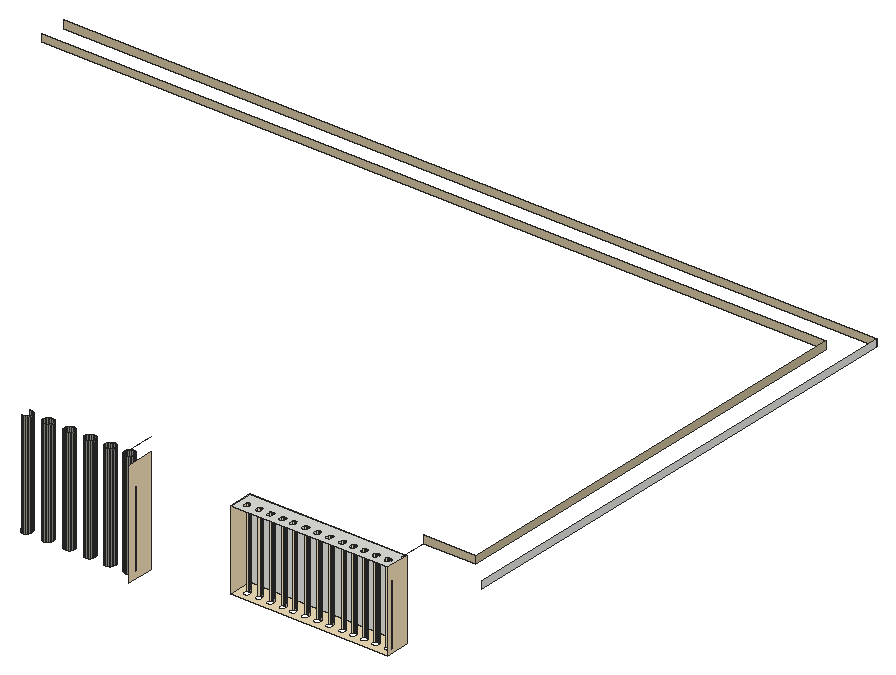
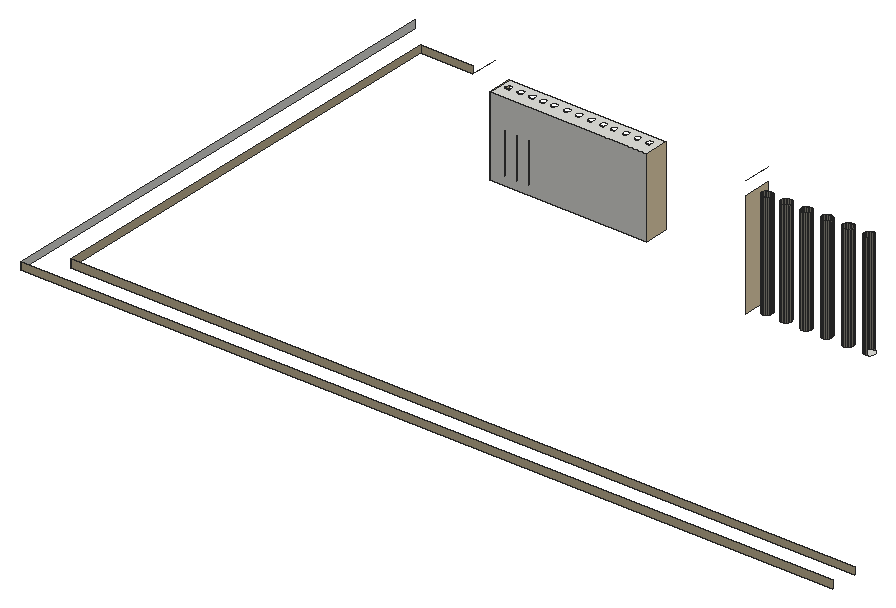
# SketchUp Ruby script. Lengths in inches.
U = 1.inch
M = Sketchup.active_model
def pt(a) = Geom::Point3d.new(a.map { |v| v * U })
def face(e, loops, mat)
  f = e.add_face(loops[0].map { |a| pt(a) })
  loops[1..].each { |l| e.add_face(l.map { |a| pt(a) }).erase! }
  f.material = f.back_material = mat if mat
  f
end
# faces: each face lists its corners as indices into pts; further lists are holes
def faces(e, pts, list, mat = nil) = list.each { |f| face(e, (f[0].is_a?(Array) ? f : [f]).map { |l| l.map { |i| pts[i] } }, mat) }
# xy, xz, yz: faces in a plane at the given z, y or x. An outline is a flat list of corners, or four numbers for a rectangle; further outlines are holes
def ring(l) = l.size == 4 ? [[l[0], l[1]], [l[2], l[1]], [l[2], l[3]], [l[0], l[3]]] : l.each_slice(2).to_a
def flat(e, list, mat, &to3) = list.each { |f| face(e, (f[0].is_a?(Array) ? f : [f]).map { |l| ring(l).map { |u, v| to3.(u, v) } }, mat) }
def xy(e, z, list, mat = nil) = flat(e, list, mat) { |x, y| [x, y, z] }
def xz(e, y, list, mat = nil) = flat(e, list, mat) { |x, z| [x, y, z] }
def yz(e, x, list, mat = nil) = flat(e, list, mat) { |y, z| [x, y, z] }
def lines(e, pts, list) = list.each { |a, b| e.add_line(pt(pts[a]), pt(pts[b])) }
# prism: a flat outline (further loops are holes) pulled along v
def prism(e, loops, v, mat = nil)
  f = face(e, loops, mat); d = Geom::Vector3d.new(v.map { |x| x * U })
  f.pushpull(f.normal.samedirection?(d) ? d.length : -d.length)
end
def box(e, o, s, mat = nil) = prism(e, [[o, [o[0] + s[0], o[1], o[2]], [o[0] + s[0], o[1] + s[1], o[2]], [o[0], o[1] + s[1], o[2]]]], [0, 0, s[2]], mat)
def at(x, y, z, deg = 0) = Geom::Transformation.translation(pt([x, y, z])) * Geom::Transformation.rotation(ORIGIN, Z_AXIS, deg.degrees)
def axes(o, x, y, z) = Geom::Transformation.new([*x, 0, *y, 0, *z, 0, *pt(o).to_a, 1])
def part(name) = M.definitions.add(name)
# library, detail: a bought-in or finely detailed component or shape, given as its bounding box
def library(name, o, s) = part(name).tap { |d| box(d.entities, o, s) }
def detail(e, o, s) = box(e.add_group.entities, o, s)
def put(e, d, t, mat = nil) = e.add_instance(d, t).tap { |i| i.material = mat if mat }
def group(e, t, mat = nil) = e.add_group.tap { |g| g.transformation = t; g.material = mat if mat }.entities
root = M.entities
M.materials.add("[Formica Graystone]").color = [149, 146, 135]
M.materials.add("[Quartz Light Brown]").color = [242, 223, 185]
M.materials.add("[Quartz Light Brown]2").color = [199, 184, 152]
xy(root,552.75,[[371.75,21.93,371.04,22.02,370.375,22.3,369.81,22.74,369.37,23.3,369.09,23.97,369,24.68,369.09,25.39,369.37,26.05,369.81,26.625,370.375,27.0625,371.04,27.34,371.75,27.43,372.46,27.34,373.125,27.0625,373.69,26.625,374.13,26.05,374.41,25.39,374.5,24.68,374.41,23.97,374.13,23.3,373.69,22.74,373.125,22.3,372.46,22.02],[383.125,21.93,382.41,22.02,381.75,22.3,381.18,22.74,380.74,23.3,380.47,23.97,380.375,24.68,380.47,25.39,380.74,26.05,381.18,26.625,381.75,27.0625,382.41,27.34,383.125,27.43,383.84,27.34,384.5,27.0625,385.07,26.625,385.51,26.05,385.78,25.39,385.875,24.68,385.78,23.97,385.51,23.3,385.07,22.74,384.5,22.3,383.84,22.02],[394.5,21.93,393.79,22.02,393.125,22.3,392.56,22.74,392.12,23.3,391.84,23.97,391.75,24.68,391.84,25.39,392.12,26.05,392.56,26.625,393.125,27.0625,393.79,27.34,394.5,27.43,395.21,27.34,395.875,27.0625,396.44,26.625,396.88,26.05,397.16,25.39,397.25,24.68,397.16,23.97,396.88,23.3,396.44,22.74,395.875,22.3,395.21,22.02],[405.3125,21.93,404.6,22.02,403.9375,22.3,403.37,22.74,402.93,23.3,402.66,23.97,402.5625,24.68,402.66,25.39,402.93,26.05,403.37,26.625,403.9375,27.0625,404.6,27.34,405.3125,27.43,406.02,27.34,406.6875,27.0625,407.26,26.625,407.69,26.05,407.97,25.39,408.0625,24.68,407.97,23.97,407.69,23.3,407.26,22.74,406.6875,22.3,406.02,22.02],[416.125,21.93,415.41,22.02,414.75,22.3,414.18,22.74,413.74,23.3,413.47,23.97,413.375,24.68,413.47,25.39,413.74,26.05,414.18,26.625,414.75,27.0625,415.41,27.34,416.125,27.43,416.84,27.34,417.5,27.0625,418.07,26.625,418.51,26.05,418.78,25.39,418.875,24.68,418.78,23.97,418.51,23.3,418.07,22.74,417.5,22.3,416.84,22.02],
  [426.375,21.93,425.66,22.02,425,22.3,424.43,22.74,423.99,23.3,423.72,23.97,423.625,24.68,423.72,25.39,423.99,26.05,424.43,26.625,425,27.0625,425.66,27.34,426.375,27.43,427.09,27.34,427.75,27.0625,428.32,26.625,428.76,26.05,429.03,25.39,429.125,24.68,429.03,23.97,428.76,23.3,428.32,22.74,427.75,22.3,427.09,22.02]])
xy(root,566.75,[[[486.91,16.1875,570.41,28.875],[504.26,18.95,503.8,19.01,503.38,19.18,503.02,19.46,502.74,19.83,502.57,20.25,502.51,20.7,502.57,21.15,502.74,21.58,503.02,21.9375,503.38,22.22,503.8,22.39,504.26,22.45,504.71,22.39,505.13,22.22,505.49,21.9375,505.77,21.58,505.95,21.15,506.01,20.7,505.95,20.25,505.77,19.83,505.49,19.46,505.13,19.18,504.71,19.01],[491.82,18.95,491.37,19.01,490.94,19.18,490.58,19.46,490.3,19.83,490.13,20.25,490.07,20.7,490.13,21.15,490.3,21.58,490.58,21.9375,490.94,22.22,491.37,22.39,491.82,22.45,492.27,22.39,492.69,22.22,493.06,21.9375,493.33,21.58,493.51,21.15,493.57,20.7,493.51,20.25,493.33,19.83,493.06,19.46,492.69,19.18,492.27,19.01],[566.44,18.95,565.99,19.01,565.57,19.18,565.21,19.46,564.93,19.83,564.75,20.25,564.69,20.7,564.75,21.15,564.93,21.58,565.21,21.9375,565.57,22.22,565.99,22.39,566.44,22.45,566.9,22.39,567.32,22.22,567.68,21.9375,567.96,21.58,568.13,21.15,568.19,20.7,568.13,20.25,567.96,19.83,567.68,19.46,567.32,19.18,566.9,19.01],[498.13,18.95,497.68,19.01,497.26,19.18,496.89,19.46,496.62,19.83,496.44,20.25,496.38,20.7,496.44,21.15,496.62,21.58,496.89,21.9375,497.26,22.22,497.68,22.39,498.13,22.45,498.58,22.39,499.01,22.22,499.37,21.9375,499.65,21.58,499.82,21.15,499.88,20.7,499.82,20.25,499.65,19.83,499.37,19.46,499.01,19.18,498.58,19.01],[560.07,18.95,559.62,19.01,559.19,19.18,558.83,19.46,558.55,19.83,558.38,20.25,558.32,20.7,558.38,21.15,558.55,21.58,558.83,21.9375,559.19,22.22,559.62,22.39,560.07,22.45,560.52,22.39,560.94,22.22,561.31,21.9375,561.58,21.58,561.76,21.15,561.82,20.7,561.76,20.25,561.58,19.83,561.31,19.46,560.94,19.18,560.52,19.01],[554.01,18.95,553.55,19.01,553.13,19.18,552.77,19.46,552.49,19.83,552.32,20.25,552.26,20.7,552.32,21.15,552.49,21.58,552.77,21.9375,553.13,22.22,553.55,22.39,554.01,22.45,554.46,22.39,554.88,22.22,555.24,21.9375,555.52,21.58,555.7,21.15,555.76,20.7,555.7,20.25,555.52,19.83,555.24,19.46,554.88,19.18,554.46,19.01],[510.69,18.95,510.24,19.01,509.82,19.18,509.46,19.46,509.18,19.83,509,20.25,508.94,20.7,509,21.15,509.18,21.58,509.46,21.9375,509.82,22.22,510.24,22.39,510.69,22.45,511.15,22.39,511.57,22.22,511.93,21.9375,512.21,21.58,512.38,21.15,512.44,20.7,512.38,20.25,512.21,19.83,511.93,19.46,511.57,19.18,511.15,19.01],[548.19,18.95,547.74,19.01,547.32,19.18,546.96,19.46,546.68,19.83,546.5,20.25,546.44,20.7,546.5,21.15,546.68,21.58,546.96,21.9375,547.32,22.22,547.74,22.39,548.19,22.45,548.65,22.39,549.07,22.22,549.43,21.9375,549.71,21.58,549.88,21.15,549.94,20.7,549.88,20.25,549.71,19.83,549.43,19.46,549.07,19.18,548.65,19.01],[529.26,18.95,528.8,19.01,528.38,19.18,528.02,19.46,527.74,19.83,527.57,20.25,527.51,20.7,527.57,21.15,527.74,21.58,528.02,21.9375,528.38,22.22,528.8,22.39,529.26,22.45,529.71,22.39,530.13,22.22,530.49,21.9375,530.77,21.58,530.95,21.15,531.01,20.7,530.95,20.25,530.77,19.83,530.49,19.46,530.13,19.18,529.71,19.01],[542.38,18.95,541.93,19.01,541.51,19.18,541.14,19.46,540.87,19.83,540.69,20.25,540.63,20.7,540.69,21.15,540.87,21.58,541.14,21.9375,541.51,22.22,541.93,22.39,542.38,22.45,542.83,22.39,543.26,22.22,543.62,21.9375,543.9,21.58,544.07,21.15,544.13,20.7,544.07,20.25,543.9,19.83,543.62,19.46,543.26,19.18,542.83,19.01],[522.82,18.95,522.37,19.01,521.94,19.18,521.58,19.46,521.3,19.83,521.13,20.25,521.07,20.7,521.13,21.15,521.3,21.58,521.58,21.9375,521.94,22.22,522.37,22.39,522.82,22.45,523.27,22.39,523.69,22.22,524.06,21.9375,524.33,21.58,524.51,21.15,524.57,20.7,524.51,20.25,524.33,19.83,524.06,19.46,523.69,19.18,523.27,19.01],[535.57,18.95,535.12,19.01,534.69,19.18,534.33,19.46,534.05,19.83,533.88,20.25,533.82,20.7,533.88,21.15,534.05,21.58,534.33,21.9375,534.69,22.22,535.12,22.39,535.57,22.45,536.02,22.39,536.44,22.22,536.81,21.9375,537.08,21.58,537.26,21.15,537.32,20.7,537.26,20.25,537.08,19.83,536.81,19.46,536.44,19.18,536.02,19.01],[516.32,18.95,515.87,19.01,515.44,19.18,515.08,19.46,514.8,19.83,514.63,20.25,514.57,20.7,514.63,21.15,514.8,21.58,515.08,21.9375,515.44,22.22,515.87,22.39,516.32,22.45,516.77,22.39,517.19,22.22,517.56,21.9375,517.83,21.58,518.01,21.15,518.07,20.7,518.01,20.25,517.83,19.83,517.56,19.46,517.19,19.18,516.77,19.01]]],"[Quartz Light Brown]")
xy(root,608.75,[[[486.91,16.1875,570.41,28.875],[516.32,18.95,516.77,19.01,517.19,19.18,517.56,19.46,517.83,19.83,518.01,20.25,518.07,20.7,518.01,21.15,517.83,21.58,517.56,21.9375,517.19,22.22,516.77,22.39,516.32,22.45,515.87,22.39,515.44,22.22,515.08,21.9375,514.8,21.58,514.63,21.15,514.57,20.7,514.63,20.25,514.8,19.83,515.08,19.46,515.44,19.18,515.87,19.01],[510.69,18.95,511.15,19.01,511.57,19.18,511.93,19.46,512.21,19.83,512.38,20.25,512.44,20.7,512.38,21.15,512.21,21.58,511.93,21.9375,511.57,22.22,511.15,22.39,510.69,22.45,510.24,22.39,509.82,22.22,509.46,21.9375,509.18,21.58,509,21.15,508.94,20.7,509,20.25,509.18,19.83,509.46,19.46,509.82,19.18,510.24,19.01],[542.38,18.95,542.83,19.01,543.26,19.18,543.62,19.46,543.9,19.83,544.07,20.25,544.13,20.7,544.07,21.15,543.9,21.58,543.62,21.9375,543.26,22.22,542.83,22.39,542.38,22.45,541.93,22.39,541.51,22.22,541.14,21.9375,540.87,21.58,540.69,21.15,540.63,20.7,540.69,20.25,540.87,19.83,541.14,19.46,541.51,19.18,541.93,19.01],[535.57,18.95,536.02,19.01,536.44,19.18,536.81,19.46,537.08,19.83,537.26,20.25,537.32,20.7,537.26,21.15,537.08,21.58,536.81,21.9375,536.44,22.22,536.02,22.39,535.57,22.45,535.12,22.39,534.69,22.22,534.33,21.9375,534.05,21.58,533.88,21.15,533.82,20.7,533.88,20.25,534.05,19.83,534.33,19.46,534.69,19.18,535.12,19.01],[504.26,18.95,504.71,19.01,505.13,19.18,505.49,19.46,505.77,19.83,505.95,20.25,506.01,20.7,505.95,21.15,505.77,21.58,505.49,21.9375,505.13,22.22,504.71,22.39,504.26,22.45,503.8,22.39,503.38,22.22,503.02,21.9375,502.74,21.58,502.57,21.15,502.51,20.7,502.57,20.25,502.74,19.83,503.02,19.46,503.38,19.18,503.8,19.01],[522.82,18.95,523.27,19.01,523.69,19.18,524.06,19.46,524.33,19.83,524.51,20.25,524.57,20.7,524.51,21.15,524.33,21.58,524.06,21.9375,523.69,22.22,523.27,22.39,522.82,22.45,522.37,22.39,521.94,22.22,521.58,21.9375,521.3,21.58,521.13,21.15,521.07,20.7,521.13,20.25,521.3,19.83,521.58,19.46,521.94,19.18,522.37,19.01],[566.44,18.95,566.9,19.01,567.32,19.18,567.68,19.46,567.96,19.83,568.13,20.25,568.19,20.7,568.13,21.15,567.96,21.58,567.68,21.9375,567.32,22.22,566.9,22.39,566.44,22.45,565.99,22.39,565.57,22.22,565.21,21.9375,564.93,21.58,564.75,21.15,564.69,20.7,564.75,20.25,564.93,19.83,565.21,19.46,565.57,19.18,565.99,19.01],[560.07,18.95,560.52,19.01,560.94,19.18,561.31,19.46,561.58,19.83,561.76,20.25,561.82,20.7,561.76,21.15,561.58,21.58,561.31,21.9375,560.94,22.22,560.52,22.39,560.07,22.45,559.62,22.39,559.19,22.22,558.83,21.9375,558.55,21.58,558.38,21.15,558.32,20.7,558.38,20.25,558.55,19.83,558.83,19.46,559.19,19.18,559.62,19.01],[554.01,18.95,554.46,19.01,554.88,19.18,555.24,19.46,555.52,19.83,555.7,20.25,555.76,20.7,555.7,21.15,555.52,21.58,555.24,21.9375,554.88,22.22,554.46,22.39,554.01,22.45,553.55,22.39,553.13,22.22,552.77,21.9375,552.49,21.58,552.32,21.15,552.26,20.7,552.32,20.25,552.49,19.83,552.77,19.46,553.13,19.18,553.55,19.01],[548.19,18.95,548.65,19.01,549.07,19.18,549.43,19.46,549.71,19.83,549.88,20.25,549.94,20.7,549.88,21.15,549.71,21.58,549.43,21.9375,549.07,22.22,548.65,22.39,548.19,22.45,547.74,22.39,547.32,22.22,546.96,21.9375,546.68,21.58,546.5,21.15,546.44,20.7,546.5,20.25,546.68,19.83,546.96,19.46,547.32,19.18,547.74,19.01],[491.82,18.95,492.27,19.01,492.69,19.18,493.06,19.46,493.33,19.83,493.51,20.25,493.57,20.7,493.51,21.15,493.33,21.58,493.06,21.9375,492.69,22.22,492.27,22.39,491.82,22.45,491.37,22.39,490.94,22.22,490.58,21.9375,490.3,21.58,490.13,21.15,490.07,20.7,490.13,20.25,490.3,19.83,490.58,19.46,490.94,19.18,491.37,19.01],[498.13,18.95,498.58,19.01,499.01,19.18,499.37,19.46,499.65,19.83,499.82,20.25,499.88,20.7,499.82,21.15,499.65,21.58,499.37,21.9375,499.01,22.22,498.58,22.39,498.13,22.45,497.68,22.39,497.26,22.22,496.89,21.9375,496.62,21.58,496.44,21.15,496.38,20.7,496.44,20.25,496.62,19.83,496.89,19.46,497.26,19.18,497.68,19.01],[529.26,18.95,529.71,19.01,530.13,19.18,530.49,19.46,530.77,19.83,530.95,20.25,531.01,20.7,530.95,21.15,530.77,21.58,530.49,21.9375,530.13,22.22,529.71,22.39,529.26,22.45,528.8,22.39,528.38,22.22,528.02,21.9375,527.74,21.58,527.57,21.15,527.51,20.7,527.57,20.25,527.74,19.83,528.02,19.46,528.38,19.18,528.8,19.01]]])
xz(root,28.875,[[486.91,566.75,570.41,608.75]])
xz(root,31.11,[[577.38,616,605.2,619.9375]],"[Quartz Light Brown]2")
xz(root,263.56,[[188.57,616,605.2,619.9375]],"[Quartz Light Brown]2")
xz(root,278.48,[[188.57,616,620.12,619.9375]],"[Quartz Light Brown]2")
yz(root,432.54,[[16.1875,552.75,31.11,608.75]],"[Quartz Light Brown]")
yz(root,486.91,[[16.1875,566.75,28.875,608.75]],"[Quartz Light Brown]")
yz(root,570.41,[[16.1875,566.75,28.875,608.75]],"[Quartz Light Brown]")
yz(root,605.2,[[31.11,616,263.56,619.9375]],"[Quartz Light Brown]2")
yz(root,620.12,[[16.1875,616,278.48,619.9375]])
p = [[371.04,22.02,552.75],[371.75,21.93,552.75],[371.75,21.93,608.75],[371.04,22.02,608.75],[372.46,22.02,552.75],[372.46,22.02,608.75],
  [382.41,22.02,552.75],[383.125,21.93,552.75],[383.125,21.93,608.75],[382.41,22.02,608.75],[383.84,22.02,552.75],[383.84,22.02,608.75],
  [393.79,22.02,552.75],[394.5,21.93,552.75],[394.5,21.93,608.75],[393.79,22.02,608.75],[395.21,22.02,552.75],[395.21,22.02,608.75],
  [404.6,22.02,552.75],[405.3125,21.93,552.75],[405.3125,21.93,608.75],[404.6,22.02,608.75],[406.02,22.02,552.75],[406.02,22.02,608.75],
  [415.41,22.02,552.75],[416.125,21.93,552.75],[416.125,21.93,608.75],[415.41,22.02,608.75],[416.84,22.02,552.75],[416.84,22.02,608.75],
  [425.66,22.02,552.75],[426.375,21.93,552.75],[426.375,21.93,608.75],[425.66,22.02,608.75],[427.09,22.02,552.75],[427.09,22.02,608.75],
  [373.125,22.3,552.75],[373.125,22.3,608.75],[381.75,22.3,552.75],[381.75,22.3,608.75],[384.5,22.3,552.75],[384.5,22.3,608.75],
  [393.125,22.3,552.75],[393.125,22.3,608.75],[395.875,22.3,552.75],[395.875,22.3,608.75],[403.9375,22.3,552.75],[403.9375,22.3,608.75],
  [406.6875,22.3,552.75],[406.6875,22.3,608.75],[414.75,22.3,552.75],[414.75,22.3,608.75],[417.5,22.3,552.75],[417.5,22.3,608.75],
  [425,22.3,552.75],[425,22.3,608.75],[427.75,22.3,552.75],[427.75,22.3,608.75],[373.69,22.74,552.75],[373.69,22.74,608.75],
  [381.18,22.74,552.75],[381.18,22.74,608.75],[385.07,22.74,552.75],[385.07,22.74,608.75],[392.56,22.74,552.75],[392.56,22.74,608.75],
  [396.44,22.74,552.75],[396.44,22.74,608.75],[403.37,22.74,552.75],[403.37,22.74,608.75],[407.26,22.74,552.75],[407.26,22.74,608.75],
  [414.18,22.74,552.75],[414.18,22.74,608.75],[418.07,22.74,552.75],[418.07,22.74,608.75],[424.43,22.74,552.75],[424.43,22.74,608.75],
  [428.32,22.74,552.75],[428.32,22.74,608.75],[374.13,23.3,552.75],[374.13,23.3,608.75],[380.74,23.3,552.75],[380.74,23.3,608.75],
  [385.51,23.3,552.75],[385.51,23.3,608.75],[392.12,23.3,552.75],[392.12,23.3,608.75],[396.88,23.3,552.75],[396.88,23.3,608.75],
  [402.93,23.3,552.75],[402.93,23.3,608.75],[407.69,23.3,552.75],[407.69,23.3,608.75],[413.74,23.3,552.75],[413.74,23.3,608.75],
  [418.51,23.3,552.75],[418.51,23.3,608.75],[423.99,23.3,552.75],[423.99,23.3,608.75],[428.76,23.3,552.75],[428.76,23.3,608.75],
  [374.41,23.97,552.75],[374.41,23.97,608.75],[380.47,23.97,552.75],[380.47,23.97,608.75],[385.78,23.97,552.75],[385.78,23.97,608.75],
  [391.84,23.97,552.75],[391.84,23.97,608.75],[397.16,23.97,552.75],[397.16,23.97,608.75],[402.66,23.97,552.75],[402.66,23.97,608.75],
  [407.97,23.97,552.75],[407.97,23.97,608.75],[413.47,23.97,552.75],[413.47,23.97,608.75],[418.78,23.97,552.75],[418.78,23.97,608.75],
  [423.72,23.97,552.75],[423.72,23.97,608.75],[429.03,23.97,552.75],[429.03,23.97,608.75],[374.5,24.68,552.75],[374.5,24.68,608.75],
  [380.375,24.68,552.75],[380.375,24.68,608.75],[385.875,24.68,552.75],[385.875,24.68,608.75],[391.75,24.68,552.75],[391.75,24.68,608.75],
  [397.25,24.68,552.75],[397.25,24.68,608.75],[402.5625,24.68,552.75],[402.5625,24.68,608.75],[408.0625,24.68,552.75],[408.0625,24.68,608.75],
  [413.375,24.68,552.75],[413.375,24.68,608.75],[418.875,24.68,552.75],[418.875,24.68,608.75],[423.625,24.68,552.75],[423.625,24.68,608.75],
  [429.125,24.68,552.75],[429.125,24.68,608.75],[374.41,25.39,552.75],[374.41,25.39,608.75],[380.47,25.39,552.75],[380.47,25.39,608.75],
  [385.78,25.39,552.75],[385.78,25.39,608.75],[391.84,25.39,552.75],[391.84,25.39,608.75],[397.16,25.39,552.75],[397.16,25.39,608.75],
  [402.66,25.39,552.75],[402.66,25.39,608.75],[407.97,25.39,552.75],[407.97,25.39,608.75],[413.47,25.39,552.75],[413.47,25.39,608.75],
  [418.78,25.39,552.75],[418.78,25.39,608.75],[423.72,25.39,552.75],[423.72,25.39,608.75],[429.03,25.39,552.75],[429.03,25.39,608.75],
  [374.13,26.05,552.75],[374.13,26.05,608.75],[380.74,26.05,552.75],[380.74,26.05,608.75],[385.51,26.05,552.75],[385.51,26.05,608.75],
  [392.12,26.05,552.75],[392.12,26.05,608.75],[396.88,26.05,552.75],[396.88,26.05,608.75],[402.93,26.05,552.75],[402.93,26.05,608.75],
  [407.69,26.05,552.75],[407.69,26.05,608.75],[413.74,26.05,552.75],[413.74,26.05,608.75],[418.51,26.05,552.75],[418.51,26.05,608.75],
  [423.99,26.05,552.75],[423.99,26.05,608.75],[428.76,26.05,552.75],[428.76,26.05,608.75],[373.69,26.625,552.75],[373.69,26.625,608.75],
  [381.18,26.625,552.75],[381.18,26.625,608.75],[385.07,26.625,552.75],[385.07,26.625,608.75],[392.56,26.625,552.75],[392.56,26.625,608.75],
  [396.44,26.625,552.75],[396.44,26.625,608.75],[403.37,26.625,552.75],[403.37,26.625,608.75],[407.26,26.625,552.75],[407.26,26.625,608.75],
  [414.18,26.625,552.75],[414.18,26.625,608.75],[418.07,26.625,552.75],[418.07,26.625,608.75],[424.43,26.625,552.75],[424.43,26.625,608.75],
  [428.32,26.625,552.75],[428.32,26.625,608.75],[373.125,27.0625,552.75],[373.125,27.0625,608.75],[381.75,27.0625,552.75],[381.75,27.0625,608.75],
  [384.5,27.0625,552.75],[384.5,27.0625,608.75],[393.125,27.0625,552.75],[393.125,27.0625,608.75],[395.875,27.0625,552.75],[395.875,27.0625,608.75],
  [403.9375,27.0625,552.75],[403.9375,27.0625,608.75],[406.6875,27.0625,552.75],[406.6875,27.0625,608.75],[414.75,27.0625,552.75],[414.75,27.0625,608.75],
  [417.5,27.0625,552.75],[417.5,27.0625,608.75],[425,27.0625,552.75],[425,27.0625,608.75],[427.75,27.0625,552.75],[427.75,27.0625,608.75],
  [372.46,27.34,552.75],[372.46,27.34,608.75],[382.41,27.34,552.75],[382.41,27.34,608.75],[383.84,27.34,552.75],[383.84,27.34,608.75],
  [393.79,27.34,552.75],[393.79,27.34,608.75],[395.21,27.34,552.75],[395.21,27.34,608.75],[404.6,27.34,552.75],[404.6,27.34,608.75],
  [406.02,27.34,552.75],[406.02,27.34,608.75],[415.41,27.34,552.75],[415.41,27.34,608.75],[416.84,27.34,552.75],[416.84,27.34,608.75],
  [425.66,27.34,552.75],[425.66,27.34,608.75],[427.09,27.34,552.75],[427.09,27.34,608.75],[371.75,27.43,552.75],[371.04,27.34,552.75],
  [371.04,27.34,608.75],[371.75,27.43,608.75],[383.125,27.43,552.75],[383.125,27.43,608.75],[394.5,27.43,552.75],[394.5,27.43,608.75],
  [405.3125,27.43,552.75],[405.3125,27.43,608.75],[416.125,27.43,552.75],[416.125,27.43,608.75],[426.375,27.43,552.75],[426.375,27.43,608.75],
  [543.9,21.58,566.75],[543.62,21.9375,566.75],[543.62,21.9375,608.75],[543.9,21.58,608.75],[546.96,21.9375,566.75],[546.68,21.58,566.75],
  [546.68,21.58,608.75],[546.96,21.9375,608.75],[549.71,21.58,566.75],[549.43,21.9375,566.75],[549.43,21.9375,608.75],[549.71,21.58,608.75],
  [552.77,21.9375,566.75],[552.49,21.58,566.75],[552.49,21.58,608.75],[552.77,21.9375,608.75],[555.52,21.58,566.75],[555.24,21.9375,566.75],
  [555.24,21.9375,608.75],[555.52,21.58,608.75],[558.83,21.9375,566.75],[558.55,21.58,566.75],[558.55,21.58,608.75],[558.83,21.9375,608.75],
  [561.58,21.58,566.75],[561.31,21.9375,566.75],[561.31,21.9375,608.75],[561.58,21.58,608.75],[565.21,21.9375,566.75],[564.93,21.58,566.75],
  [564.93,21.58,608.75],[565.21,21.9375,608.75],[567.96,21.58,566.75],[567.68,21.9375,566.75],[567.68,21.9375,608.75],[567.96,21.58,608.75],
  [490.94,22.22,566.75],[490.58,21.9375,566.75],[490.58,21.9375,608.75],[490.94,22.22,608.75],[493.06,21.9375,566.75],[492.69,22.22,566.75],
  [492.69,22.22,608.75],[493.06,21.9375,608.75],[497.26,22.22,566.75],[496.89,21.9375,566.75],[496.89,21.9375,608.75],[497.26,22.22,608.75],
  [499.37,21.9375,566.75],[499.01,22.22,566.75],[499.01,22.22,608.75],[499.37,21.9375,608.75],[503.38,22.22,566.75],[503.02,21.9375,566.75],
  [503.02,21.9375,608.75],[503.38,22.22,608.75],[505.49,21.9375,566.75],[505.13,22.22,566.75],[505.13,22.22,608.75],[505.49,21.9375,608.75],
  [509.82,22.22,566.75],[509.46,21.9375,566.75],[509.46,21.9375,608.75],[509.82,22.22,608.75],[511.93,21.9375,566.75],[511.57,22.22,566.75],
  [511.57,22.22,608.75],[511.93,21.9375,608.75],[515.44,22.22,566.75],[515.08,21.9375,566.75],[515.08,21.9375,608.75],[515.44,22.22,608.75],
  [517.56,21.9375,566.75],[517.19,22.22,566.75],[517.19,22.22,608.75],[517.56,21.9375,608.75],[521.94,22.22,566.75],[521.58,21.9375,566.75],
  [521.58,21.9375,608.75],[521.94,22.22,608.75],[524.06,21.9375,566.75],[523.69,22.22,566.75],[523.69,22.22,608.75],[524.06,21.9375,608.75],
  [528.38,22.22,566.75],[528.02,21.9375,566.75],[528.02,21.9375,608.75],[528.38,22.22,608.75],[530.49,21.9375,566.75],[530.13,22.22,566.75],
  [530.13,22.22,608.75],[530.49,21.9375,608.75],[534.69,22.22,566.75],[534.33,21.9375,566.75],[534.33,21.9375,608.75],[534.69,22.22,608.75],
  [536.81,21.9375,566.75],[536.44,22.22,566.75],[536.44,22.22,608.75],[536.81,21.9375,608.75],[541.51,22.22,566.75],[541.14,21.9375,566.75],
  [541.14,21.9375,608.75],[541.51,22.22,608.75],[543.26,22.22,566.75],[543.26,22.22,608.75],[547.32,22.22,566.75],[547.32,22.22,608.75],
  [549.07,22.22,566.75],[549.07,22.22,608.75],[553.13,22.22,566.75],[553.13,22.22,608.75],[554.88,22.22,566.75],[554.88,22.22,608.75],
  [559.19,22.22,566.75],[559.19,22.22,608.75],[560.94,22.22,566.75],[560.94,22.22,608.75],[565.57,22.22,566.75],[565.57,22.22,608.75],
  [567.32,22.22,566.75],[567.32,22.22,608.75],[491.37,22.39,566.75],[491.37,22.39,608.75],[492.27,22.39,566.75],[492.27,22.39,608.75],
  [497.68,22.39,566.75],[497.68,22.39,608.75],[498.58,22.39,566.75],[498.58,22.39,608.75],[503.8,22.39,566.75],[503.8,22.39,608.75],
  [504.71,22.39,566.75],[504.71,22.39,608.75],[510.24,22.39,566.75],[510.24,22.39,608.75],[511.15,22.39,566.75],[511.15,22.39,608.75],
  [515.87,22.39,566.75],[515.87,22.39,608.75],[516.77,22.39,566.75],[516.77,22.39,608.75],[522.37,22.39,566.75],[522.37,22.39,608.75],
  [523.27,22.39,566.75],[523.27,22.39,608.75],[528.8,22.39,566.75],[528.8,22.39,608.75],[529.71,22.39,566.75],[529.71,22.39,608.75],
  [535.12,22.39,566.75],[535.12,22.39,608.75],[536.02,22.39,566.75],[536.02,22.39,608.75],[541.93,22.39,566.75],[541.93,22.39,608.75],
  [542.83,22.39,566.75],[542.83,22.39,608.75],[547.74,22.39,566.75],[547.74,22.39,608.75],[548.65,22.39,566.75],[548.65,22.39,608.75],
  [553.55,22.39,566.75],[553.55,22.39,608.75],[554.46,22.39,566.75],[554.46,22.39,608.75],[559.62,22.39,566.75],[559.62,22.39,608.75],
  [560.52,22.39,566.75],[560.52,22.39,608.75],[565.99,22.39,566.75],[565.99,22.39,608.75],[566.9,22.39,566.75],[566.9,22.39,608.75],
  [491.82,22.45,566.75],[491.82,22.45,608.75],[498.13,22.45,566.75],[498.13,22.45,608.75],[504.26,22.45,566.75],[504.26,22.45,608.75],
  [510.69,22.45,566.75],[510.69,22.45,608.75],[516.32,22.45,566.75],[516.32,22.45,608.75],[522.82,22.45,566.75],[522.82,22.45,608.75],
  [529.26,22.45,566.75],[529.26,22.45,608.75],[535.57,22.45,566.75],[535.57,22.45,608.75],[542.38,22.45,566.75],[542.38,22.45,608.75],
  [548.19,22.45,566.75],[548.19,22.45,608.75],[554.01,22.45,566.75],[554.01,22.45,608.75],[560.07,22.45,566.75],[560.07,22.45,608.75],
  [566.44,22.45,566.75],[566.44,22.45,608.75],[432.54,16.1875,616],[432.54,31.11,616],[577.38,16.1875,616],[577.38,31.11,616]]
faces(root,p,[[0,1,2,3],[1,4,5,2],[6,7,8,9],[7,10,11,8],[12,13,14,15],[13,16,17,14],[18,19,20,21],[19,22,23,20],
  [24,25,26,27],[25,28,29,26],[30,31,32,33],[31,34,35,32],[4,36,37,5],[38,6,9,39],[10,40,41,11],[42,12,15,43],
  [16,44,45,17],[46,18,21,47],[22,48,49,23],[50,24,27,51],[28,52,53,29],[54,30,33,55],[34,56,57,35],[36,58,59,37],
  [60,38,39,61],[40,62,63,41],[64,42,43,65],[44,66,67,45],[68,46,47,69],[48,70,71,49],[72,50,51,73],[52,74,75,53],
  [76,54,55,77],[56,78,79,57],[58,80,81,59],[82,60,61,83],[62,84,85,63],[86,64,65,87],[66,88,89,67],[90,68,69,91],
  [70,92,93,71],[94,72,73,95],[74,96,97,75],[98,76,77,99],[78,100,101,79],[80,102,103,81],[104,82,83,105],[84,106,107,85],
  [108,86,87,109],[88,110,111,89],[112,90,91,113],[92,114,115,93],[116,94,95,117],[96,118,119,97],[120,98,99,121],[100,122,123,101],
  [102,124,125,103],[126,104,105,127],[106,128,129,107],[130,108,109,131],[110,132,133,111],[134,112,113,135],[114,136,137,115],[138,116,117,139],
  [118,140,141,119],[142,120,121,143],[122,144,145,123],[124,146,147,125],[148,126,127,149],[128,150,151,129],[152,130,131,153],[132,154,155,133],
  [156,134,135,157],[136,158,159,137],[160,138,139,161],[140,162,163,141],[164,142,143,165],[144,166,167,145],[146,168,169,147],[170,148,149,171],
  [150,172,173,151],[174,152,153,175],[154,176,177,155],[178,156,157,179],[158,180,181,159],[182,160,161,183],[162,184,185,163],[186,164,165,187],
  [166,188,189,167],[168,190,191,169],[192,170,171,193],[172,194,195,173],[196,174,175,197],[176,198,199,177],[200,178,179,201],[180,202,203,181],
  [204,182,183,205],[184,206,207,185],[208,186,187,209],[188,210,211,189],[190,212,213,191],[214,192,193,215],[194,216,217,195],[218,196,197,219],
  [198,220,221,199],[222,200,201,223],[202,224,225,203],[226,204,205,227],[206,228,229,207],[230,208,209,231],[210,232,233,211],[212,234,235,213],
  [236,214,215,237],[216,238,239,217],[240,218,219,241],[220,242,243,221],[244,222,223,245],[224,246,247,225],[248,226,227,249],[228,250,251,229],
  [252,230,231,253],[232,254,255,233],[256,257,258,259],[234,256,259,235],[260,236,237,261],[238,260,261,239],[262,240,241,263],[242,262,263,243],
  [264,244,245,265],[246,264,265,247],[266,248,249,267],[250,266,267,251],[268,252,253,269],[254,268,269,255]],"[Formica Graystone]")
faces(root,p,[[270,271,272,273],[274,275,276,277],[278,279,280,281],[282,283,284,285],[286,287,288,289],[290,291,292,293],[294,295,296,297],[298,299,300,301],
  [302,303,304,305],[306,307,308,309],[310,311,312,313],[314,315,316,317],[318,319,320,321],[322,323,324,325],[326,327,328,329],[330,331,332,333],
  [334,335,336,337],[338,339,340,341],[342,343,344,345],[346,347,348,349],[350,351,352,353],[354,355,356,357],[358,359,360,361],[362,363,364,365],
  [366,367,368,369],[370,371,372,373],[271,374,375,272],[376,274,277,377],[279,378,379,280],[380,282,285,381],[287,382,383,288],[384,290,293,385],
  [295,386,387,296],[388,298,301,389],[303,390,391,304],[392,306,309,393],[311,394,395,312],[396,314,317,397],[319,398,399,320],[400,322,325,401],
  [327,402,403,328],[404,330,333,405],[335,406,407,336],[408,338,341,409],[343,410,411,344],[412,346,349,413],[351,414,415,352],[416,354,357,417],
  [359,418,419,360],[420,362,365,421],[367,422,423,368],[424,370,373,425],[374,426,427,375],[428,376,377,429],[378,430,431,379],[432,380,381,433],
  [382,434,435,383],[436,384,385,437],[386,438,439,387],[440,388,389,441],[390,442,443,391],[444,392,393,445],[394,444,445,395],[446,396,397,447],
  [398,446,447,399],[448,400,401,449],[402,448,449,403],[450,404,405,451],[406,450,451,407],[452,408,409,453],[410,452,453,411],[454,412,413,455],
  [414,454,455,415],[456,416,417,457],[418,456,457,419],[458,420,421,459],[422,458,459,423],[460,424,425,461],[426,460,461,427],[462,428,429,463],
  [430,462,463,431],[464,432,433,465],[434,464,465,435],[466,436,437,467],[438,466,467,439],[468,440,441,469],[442,468,469,443]],"[Quartz Light Brown]")
lines(root,p,[[470,471],[472,473]])
